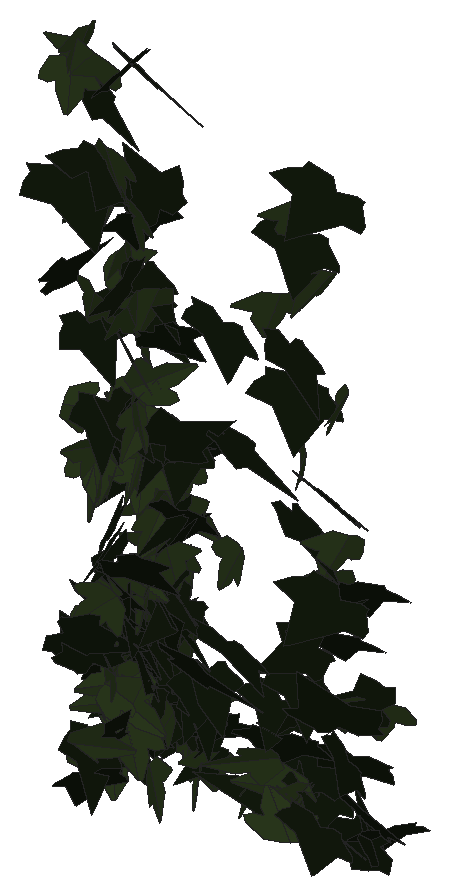
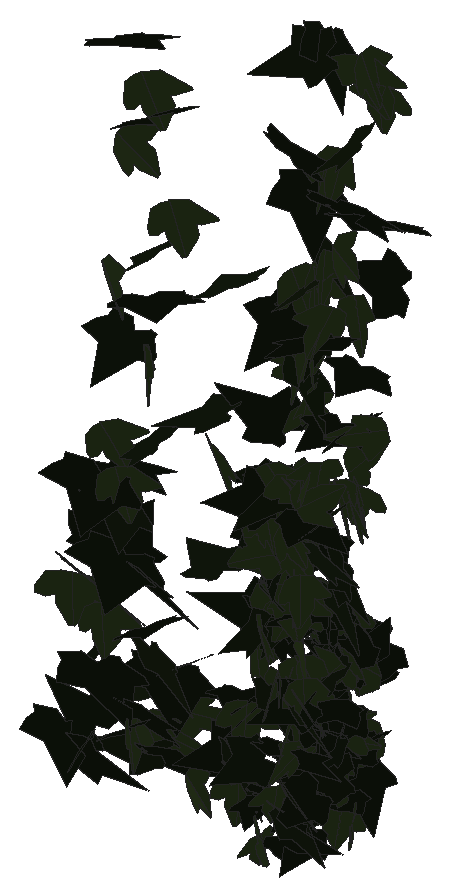
# SketchUp Ruby script. Lengths in millimetres.
U = 1.mm
M = Sketchup.active_model
def pt(a) = Geom::Point3d.new(a.map { |v| v * U })
def face(e, loops, mat)
  f = e.add_face(loops[0].map { |a| pt(a) })
  loops[1..].each { |l| e.add_face(l.map { |a| pt(a) }).erase! }
  f.material = f.back_material = mat if mat
  f
end
# faces: each face lists its corners as indices into pts; further lists are holes
def faces(e, pts, list, mat = nil) = list.each { |f| face(e, (f[0].is_a?(Array) ? f : [f]).map { |l| l.map { |i| pts[i] } }, mat) }
# xy, xz, yz: faces in a plane at the given z, y or x. An outline is a flat list of corners, or four numbers for a rectangle; further outlines are holes
def ring(l) = l.size == 4 ? [[l[0], l[1]], [l[2], l[1]], [l[2], l[3]], [l[0], l[3]]] : l.each_slice(2).to_a
def flat(e, list, mat, &to3) = list.each { |f| face(e, (f[0].is_a?(Array) ? f : [f]).map { |l| ring(l).map { |u, v| to3.(u, v) } }, mat) }
def xy(e, z, list, mat = nil) = flat(e, list, mat) { |x, y| [x, y, z] }
def xz(e, y, list, mat = nil) = flat(e, list, mat) { |x, z| [x, y, z] }
def yz(e, x, list, mat = nil) = flat(e, list, mat) { |y, z| [x, y, z] }
def lines(e, pts, list) = list.each { |a, b| e.add_line(pt(pts[a]), pt(pts[b])) }
# prism: a flat outline (further loops are holes) pulled along v
def prism(e, loops, v, mat = nil)
  f = face(e, loops, mat); d = Geom::Vector3d.new(v.map { |x| x * U })
  f.pushpull(f.normal.samedirection?(d) ? d.length : -d.length)
end
def box(e, o, s, mat = nil) = prism(e, [[o, [o[0] + s[0], o[1], o[2]], [o[0] + s[0], o[1] + s[1], o[2]], [o[0], o[1] + s[1], o[2]]]], [0, 0, s[2]], mat)
def at(x, y, z, deg = 0) = Geom::Transformation.translation(pt([x, y, z])) * Geom::Transformation.rotation(ORIGIN, Z_AXIS, deg.degrees)
def axes(o, x, y, z) = Geom::Transformation.new([*x, 0, *y, 0, *z, 0, *pt(o).to_a, 1])
def part(name) = M.definitions.add(name)
# library, detail: a bought-in or finely detailed component or shape, given as its bounding box
def library(name, o, s) = part(name).tap { |d| box(d.entities, o, s) }
def detail(e, o, s) = box(e.add_group.entities, o, s)
def put(e, d, t, mat = nil) = e.add_instance(d, t).tap { |i| i.material = mat if mat }
def group(e, t, mat = nil) = e.add_group.tap { |g| g.transformation = t; g.material = mat if mat }.entities
root = M.entities
M.materials.add("efeu1").color = [18, 25, 13]
M.materials.add("efeu2").color = [43, 57, 29]
c1 = part("ivyleaf_9")
p = [[39.1,54.8,31.7],[34.5,51.8,30.2],[-5.3,25.2,17.3],[-17.9,28.3,20.9],[-21.6,21.7,17],[-20.2,4.3,5.3],
  [-22.9,-0.3,2.5],[-17.1,-4,-0.6],[-2,-2.1,-1.2],[-0.7,-15.4,-10.1],[16.6,-22.3,-16.7],[21.1,-15.1,-12.5],
  [32.7,-10.7,-11],[46.1,-1.8,-6.6],[30.8,11.2,3.8]]
faces(c1.entities,p,[[0,1,2,3,4,5,6,7,8,9,10,11,12,13,14]],"efeu1")
c2 = part("ivyleaf_10")
p = [[0,12.8,-0.8],[-1.5,51.3,-10.9],[-4.9,51,-11.6],[-13.6,26.5,-7.3],[-13.2,15.9,-4.6],[-21.1,19.3,-7.2],
  [-29.5,16.3,-8.3],[-29.2,8.3,-6.2],[-19.7,-9.8,0.5],[-7.6,-13,4],[1,-12.2,5.8],[-0.4,51.1,-11.1],
  [-1.5,51.1,-10.9],[1,-12.4,5.9],[16.9,-12.4,3.5],[35.1,9.1,-5.1],[35,12.9,-6.1],[20.5,16.4,-4.9],
  [15.8,15,-3.8],[15.3,27.6,-7.1],[12.8,31.3,-7.8]]
faces(c2.entities,p,[[0,1,2,3,4,5,6,7,8,9,10],[11,12,0,13,14,15,16,17,18,19,20]],"efeu2")
put(root,c1,axes([736,1006.8,1673],[-0.48258,0.69438,-0.16098],[-0.11218,-0.23228,-0.77598],[-0.86235,-0.35837,0.19103]))
put(root,c2,axes([717.6,870.9,2505.8],[1.2073,0.09097,0.06116],[0.06582,0.07936,-0.99101],[-0.11642,0.9883,0.07394]))
put(root,c2,axes([725.1,886.3,2544.7],[0.09502,-1.01576,0.19504],[0.05123,-0.19232,-1.0184],[1.26083,0.08436,0.02669]))
put(root,c1,axes([731.4,969.1,1978.9],[-0.96634,0.16266,-0.36138],[0.32603,-0.37717,-0.7555],[-0.35703,-0.78469,0.28823]))
put(root,c2,axes([723.2,924.8,1838.9],[0.90491,-0.52897,-0.04758],[-0.0478,0.027,-0.91103],[0.64619,0.74277,-0.00076]))
put(root,c2,axes([729,903.9,1639.6],[0.31669,-0.47404,-0.71017],[-0.18791,0.70409,-0.52628],[1.02461,0.27564,0.12298]))
put(root,c2,axes([744.6,871.5,2527.6],[-1.64861,0.10035,0.44623],[-0.86974,-0.15074,-0.85322],[-0.03566,-0.96268,0.18012]))
put(root,c2,axes([741.3,969.4,2037.5],[-0.69821,0.05512,-0.68237],[-0.83211,-0.12231,0.56217],[-0.07175,0.88216,0.12058]))
put(root,c1,axes([737.5,997.8,1805.7],[-0.81287,0.5246,-0.03584],[0.02253,-0.03447,-0.84788],[-0.64111,-0.66636,0.01564]))
put(root,c2,axes([726.8,991.4,1824.4],[-0.46572,-0.77141,-0.05585],[0.06616,0.03544,-0.86007],[0.94126,-0.38417,0.03282]))
put(root,c1,axes([715.3,844.8,2258.7],[0.17072,0.92716,-0.37618],[-0.0976,0.38899,0.92897],[1.21678,-0.09888,0.1273]))
put(root,c1,axes([709.9,885.4,2358.7],[-0.72181,-0.79752,-0.36037],[0.82373,0.17043,-0.83269],[1.44765,-0.49463,0.29413]))
put(root,c1,axes([736.3,998.9,1741.5],[-0.89598,-0.36202,0.18741],[-0.19448,-0.10037,-0.81857],[0.45774,-0.75127,0.01905]))
put(root,c1,axes([719.8,982.7,1694.4],[0.6203,0.55737,0.33393],[0.29686,0.22982,-0.75409],[-0.735,0.56321,-0.02275]))
put(root,c2,axes([731.7,923.6,1669],[-0.64135,0.6965,-0.0657],[-0.05246,0.04986,0.87262],[0.85189,0.52744,0.00427]))
put(root,c1,axes([710.8,959,1826.5],[0.4423,-0.69829,0.3383],[0.25011,-0.27393,-0.78513],[0.91298,0.41333,0.05119]))
put(root,c1,axes([712.3,945.4,1703.4],[0.70376,0.08993,0.64163],[0.62061,0.46919,-0.52309],[-0.48953,0.72409,0.25926]))
put(root,c1,axes([742.8,1010.2,1647.9],[-0.14857,-0.20705,-0.77913],[-0.44615,-0.68805,0.24],[-0.87652,0.38531,0.0099]))
put(root,c1,axes([714,955.6,1799.8],[-0.25147,-0.40809,-0.74835],[0.60556,0.56845,-0.4467],[0.84541,-0.52857,0.09737]))
put(root,c1,axes([721.6,939.4,1741.8],[0.91558,-0.22593,-0.36094],[-0.40085,0.158,-0.78206],[0.33045,0.81764,0.05139]))
put(root,c1,axes([743.1,912.1,1894.6],[-0.39537,0.7781,0.31895],[-0.16045,0.29071,-0.84284],[-1.01331,-0.34963,0.00901]))
put(root,c2,axes([716.2,944.2,1835.7],[0.8108,0.05931,0.54121],[0.65816,0.04351,-0.66722],[-0.08963,0.85598,-0.00359]))
put(root,c2,axes([735.8,889.4,2027.4],[0.53517,-0.7577,-0.29504],[-0.14727,0.27084,-0.87502],[0.98101,0.45401,0.0296]))
put(root,c1,axes([731.9,908.8,1764.9],[0.45542,0.7726,0.26468],[0.16634,0.22798,-0.85776],[-0.98236,0.39677,-0.02254]))
put(root,c1,axes([721.4,902.1,2181.3],[-0.45284,-0.47083,-0.70904],[0.67793,0.45188,-0.59095],[0.78654,-0.66055,0.10113]))
put(root,c1,axes([717.5,910.8,2461.5],[0.79664,-0.71391,-0.19548],[-0.02365,0.24409,-0.9562],[0.90272,0.63641,0.14745]))
put(root,c1,axes([720.9,965.6,2021.5],[0.13454,-0.88447,0.1392],[0.16263,-0.12247,-0.88377],[1.08016,0.1286,0.11573]))
put(root,c1,axes([731.7,974.8,1642.6],[0.47381,0.66938,0.24934],[0.1563,0.21394,-0.77388],[-0.85733,0.40894,-0.00328]))
put(root,c2,axes([733,998.4,1745.6],[-0.01133,0.37561,0.74869],[-0.12988,0.74214,-0.37364],[-1.01362,-0.0993,0.03951]))
put(root,c1,axes([709.1,919.4,1827],[0.57125,-0.39976,0.7706],[0.80492,-0.40518,-0.61108],[0.68835,0.80555,0.07506]))
put(root,c2,axes([730.2,959.9,2080.7],[0.58265,0.77237,0.01431],[0.0084,0.01256,-0.90809],[-0.94241,0.47763,0.00075]))
put(root,c2,axes([713.5,896.6,1811],[-0.00894,0.0213,-0.94912],[1.04229,-0.41376,-0.01588],[-0.50507,-0.85421,-0.01597]))
put(root,c2,axes([728.5,927.2,1639.4],[0.88697,0.46011,0.12325],[0.12377,0.07016,-0.86037],[-0.56779,0.73405,0.00498]))
put(root,c1,axes([742.1,987.8,1815.7],[-0.87665,0.277,-0.35839],[0.4005,-0.1446,-0.76996],[-0.38076,-0.78986,0.01527]))
put(root,c1,axes([744.5,971.1,2027.2],[-0.02977,0.36675,-0.81999],[-0.02135,-0.82033,-0.36639],[-1.09568,0.00602,0.02942]))
put(root,c2,axes([751.3,913.8,1724],[-0.17277,-0.06921,0.89006],[-0.64483,-0.71976,-0.14007],[0.87774,-0.5424,0.0723]))
put(root,c1,axes([746.4,904.9,2375.2],[-1.72779,-0.27021,-0.19313],[0.42227,-0.07509,-0.93788],[0.47039,-0.92511,0.13254]))
put(root,c1,axes([743.8,877.4,1786.4],[0.63994,0.20871,0.81274],[-0.99444,-0.10086,0.55197],[0.24309,-0.96204,0.11845]))
put(root,c2,axes([750.3,876.1,2234],[-0.9863,0.21956,0.49643],[-0.58372,0.13238,-0.83773],[-0.31277,-0.93942,-0.00203]))
put(root,c1,axes([728.3,920.7,1665.8],[-0.03432,-0.26209,-0.82208],[0.09454,0.81842,-0.26357],[1.04841,-0.08238,-0.00315]))
put(root,c2,axes([743.8,914.8,1742.7],[-0.10282,0.13445,0.85306],[-0.16595,-0.84848,0.12029],[1.04042,-0.12205,0.10349]))
put(root,c2,axes([735.6,918.3,2323],[0.30207,-0.77973,0.55458],[0.22308,-0.52374,-0.81799],[1.14583,0.30752,0.01305]))
put(root,c2,axes([721.3,877.4,2092.5],[-0.12433,-0.16946,-0.90765],[0.97322,0.44367,-0.1724],[0.56724,-0.79835,0.09685]))
put(root,c2,axes([743.1,882.8,2045.8],[-0.13572,-0.17882,-0.91596],[-0.39439,-0.85796,0.20676],[-1.06808,0.33952,0.04005]))
put(root,c1,axes([744.8,903.1,1927.9],[0.09412,0.37838,0.81761],[0.03316,0.81925,-0.3817],[-1.09863,0.05715,0.05852]))
put(root,c1,axes([748.6,1000.3,1706.5],[-0.86466,0.36783,-0.19995],[0.22377,-0.0806,-0.7984],[-0.45914,-0.73198,-0.01257]))
put(root,c1,axes([723.1,991.5,1809.5],[0.97435,0.01676,0.27768],[0.33253,0.12166,-0.79129],[-0.06786,0.83674,0.10949]))
put(root,c1,axes([733,933.5,1805.6],[-0.18666,-0.79125,-0.28943],[0.08847,0.2807,-0.80573],[1.02407,-0.16847,0.01686]))
put(root,c2,axes([731.3,891,2020.8],[1.05702,0.20621,0.23006],[0.27015,0.06321,-0.89056],[-0.26285,0.8942,0.0099]))
put(root,c2,axes([736,893.7,2000.1],[0.80158,-0.60895,0.23322],[0.22443,-0.14453,-0.89564],[0.76323,0.68205,0.01844]))
put(root,c2,axes([738.8,941.5,1667.1],[-0.10905,0.44318,-0.72072],[-0.03627,-0.72593,-0.44269],[-1.03158,-0.02133,0.09175]))
put(root,c2,axes([744.1,975.5,1938.4],[-0.5166,-0.76141,-0.08895],[0.06216,0.07344,-0.87119],[0.93317,-0.4264,0.00879]))
put(root,c1,axes([749.8,904.2,1922.2],[-0.65855,0.56241,-0.45279],[0.36666,-0.33901,-0.77938],[-0.80093,-0.61762,0.0155]))
put(root,c2,axes([754.8,887.5,1858.6],[0.9417,-0.09258,-0.62262],[-0.73784,0.16407,-0.77417],[0.21291,0.97803,0.07094]))
put(root,c2,axes([745.4,987.5,1772.2],[0.16886,-0.51456,-0.6732],[0.04897,0.68534,-0.51558],[1.03258,0.05164,0.13454]))
put(root,c2,axes([736.6,913.2,1726.6],[0.93062,0.41804,0.17335],[0.1732,0.10154,-0.8696],[-0.52425,0.77563,0.02042]))
put(root,c1,axes([726.9,856,1823],[0.20086,0.2909,-0.99963],[0.42725,0.9376,0.33053],[1.19612,-0.38376,0.0498]))
put(root,c2,axes([741.3,932.4,2250.5],[0.45358,0.76775,0.46826],[-0.00721,0.50878,-0.82949],[-1.0971,0.31407,0.19905]))
put(root,c2,axes([750.3,955.8,1825.5],[-0.09574,-0.85595,-0.12657],[0.02321,0.12607,-0.85742],[1.6466,-0.05154,0.00473]))
put(root,c2,axes([760,885.6,1774.4],[0.39352,-0.132,-0.88914],[-0.57724,0.77827,-0.28718],[0.93243,0.53751,0.19746]))
put(root,c2,axes([743.9,969.3,2070.8],[-0.65818,0.69521,-0.22127],[0.16239,-0.17679,-0.87997],[-0.87514,-0.55566,0.00313]))
put(root,c2,axes([748.5,929.6,1764],[0.22728,-0.80974,0.20425],[0.08657,-0.19317,-0.83052],[1.01515,0.19776,0.02509]))
put(root,c2,axes([761.4,952.1,1839.8],[-0.07546,0.3997,0.77683],[-0.7953,0.49735,-0.3078],[-0.70957,-0.59995,0.26238]))
put(root,c1,axes([760.3,941.1,1735.7],[-0.93968,-0.30032,0.21904],[-0.23196,-0.11474,-0.8259],[0.38968,-0.79251,0.03657]))
put(root,c1,axes([758.3,856,1659.1],[0.28146,0.86352,-0.3889],[-0.24564,-0.3464,-0.88859],[-1.12899,0.29064,0.09638]))
put(root,c2,axes([747,919.3,1742.4],[-0.4042,0.80604,-0.08092],[0.0391,-0.07431,-0.87147],[-0.98753,-0.33285,-0.00139]))
put(root,c2,axes([756.8,959.6,1827.2],[-0.77078,-0.74938,0.15285],[-0.03604,-0.16308,-0.8497],[1.45514,-0.40098,0.05992]))
put(root,c2,axes([753.2,897.7,2014.7],[0.64834,-0.7488,-0.1849],[-0.09965,0.16864,-0.91771],[0.93569,0.5368,0.03038]))
put(root,c2,axes([739.9,959.8,2206.4],[0.14482,-0.36931,0.83747],[0.76007,-0.58605,-0.34675],[0.81804,0.60991,0.17392]))
put(root,c1,axes([750.7,932.8,1771.3],[0.69116,0.66139,0.01987],[0.01602,0.01492,-0.87085],[-0.8071,0.56668,-0.00027]))
put(root,c2,axes([751.6,933.6,1754.1],[0.16921,0.7117,-0.47499],[-0.10863,-0.46658,-0.72509],[-1.03823,0.16481,-0.00155]))
put(root,c2,axes([752.3,1007.2,1697.9],[0.30272,0.78233,-0.00714],[-0.02778,-0.00027,-0.82046],[-0.95408,0.24823,0.02162]))
put(root,c1,axes([755.1,939.8,1684.2],[0.89841,0.27505,-0.37064],[-0.43776,-0.09781,-0.78549],[-0.35418,0.81859,0.03069]))
put(root,c1,axes([747.5,887.5,2088.8],[-0.02216,-0.95704,0.09186],[-0.00737,-0.09176,-0.95721],[1.17294,-0.01865,-0.00428]))
put(root,c1,axes([744,881.2,1683.4],[0.81897,0.69571,0.17028],[-0.15216,-0.11627,0.96673],[0.86047,-0.68272,0.00888]))
put(root,c1,axes([749,874.3,1688.2],[-0.02427,-1.0511,0.16075],[-0.03966,-0.1601,-1.05088],[1.29664,-0.02457,-0.02914]))
put(root,c2,axes([755.9,947.2,1707.3],[0.17231,0.77284,-0.3112],[-0.05984,-0.30738,-0.78561],[-1.01467,0.14937,-0.00652]))
put(root,c1,axes([773.4,995.5,1743],[-0.96985,-0.09923,0.27915],[-0.32044,-0.13375,-0.79552],[0.16721,-0.83186,0.09461]))
put(root,c2,axes([770.5,918.5,1759.8],[0.66931,0.24639,-0.65135],[-0.77824,-0.15483,-0.59586],[-0.34082,0.83741,0.08147]))
put(root,c1,axes([767.8,904.7,1845.9],[0.09704,-0.15827,0.8892],[-0.12332,0.88547,0.16664],[-1.09495,-0.11376,0.06003]))
put(root,c1,axes([747.1,993.7,1724.1],[0.34575,-0.79481,0.06296],[0.0433,-0.05417,-0.84369],[0.97174,0.28521,0.0152]))
put(root,c1,axes([776.4,999.6,1674],[-0.93088,0.22794,0.16029],[-0.21323,-0.02753,-0.79281],[-0.26479,-0.77919,0.0749]))
put(root,c2,axes([757.3,951.6,1689.3],[0.84842,-0.46742,0.16983],[0.16462,-0.10366,-0.83785],[0.58397,0.70832,-0.01054]))
put(root,c2,axes([760.5,930.5,2008.1],[0.77871,-0.65031,0.05837],[0.05505,-0.03751,-0.91119],[0.79466,0.63985,0.00592]))
put(root,c1,axes([743.7,913.7,1860.1],[0.26242,-0.43106,0.73589],[0.62874,-0.539,-0.46637],[0.82902,0.54524,0.12076]))
put(root,c2,axes([765.4,883.6,2410.3],[-1.11871,0.40198,0.01413],[-0.0154,0.00641,-1.00121],[-0.49047,-0.91706,-0.0008]))
put(root,c2,axes([757.1,1022.2,1625.1],[0.46437,-0.65917,-0.25275],[0.16061,-0.21583,0.76115],[-0.84617,-0.40271,0.00577]))
put(root,c2,axes([749.7,851.7,1694.3],[0.3085,-0.03046,1.00775],[0.57542,0.92184,-0.09049],[-1.08712,0.47929,0.23808]))
put(root,c1,axes([748.2,960.3,1803.8],[0.35787,-0.83335,0.10377],[0.05058,-0.10038,-0.85429],[1.59748,0.18987,0.0038]))
put(root,c1,axes([755.1,920.2,1675.2],[0.34521,-0.70848,-0.43848],[-0.08918,0.44019,-0.7584],[1.01258,0.2803,0.0827]))
put(root,c1,axes([777.7,984.6,1804.6],[-0.42966,0.79212,-0.04949],[0.01828,-0.04749,-0.86686],[-0.9681,-0.35245,0.00559]))
put(root,c2,axes([767.1,987.6,1817.4],[0.25119,-0.55728,-0.63968],[0.07148,0.66601,-0.56137],[1.03255,0.08946,0.19447]))
put(root,c1,axes([775.4,935.1,1737.8],[-1.02836,-0.22041,-0.05985],[0.06915,0.01981,-0.87124],[0.26992,-0.84481,-0.00482]))
put(root,c2,axes([769.5,953.2,2041],[-1.04334,-0.32834,-0.08377],[0.0929,0.03539,-0.91604],[0.40283,-0.85856,-0.00572]))
put(root,c1,axes([758.1,932.2,1823.6],[0.06148,-0.69395,0.56336],[0.07548,-0.56019,-0.69558],[1.08786,0.07809,0.01643]))
put(root,c2,axes([765.6,1018,1640.6],[0.14264,0.77451,-0.16715],[-0.02994,-0.16534,-0.78328],[-0.96619,0.11946,-0.00041]))
put(root,c2,axes([770.5,985.5,1815.7],[-0.76645,0.60557,-0.01651],[-0.09559,-0.10481,-0.86287],[-0.73287,-0.61965,0.12982]))
put(root,c2,axes([782.4,953.9,1903.5],[-1.58601,-0.16244,0.23055],[-0.42492,-0.05944,-0.84889],[0.32796,-0.8626,0.01508]))
put(root,c2,axes([771.2,897.6,2291.6],[0.10911,-0.8559,-0.45372],[0.05165,0.45867,-0.85689],[1.18072,0.05903,0.07942]))
put(root,c2,axes([765.2,935.7,2000.8],[1.08167,0.2075,0.01562],[0.01724,0.00815,-0.91056],[-0.25328,0.88672,0.00471]))
put(root,c1,axes([754.7,927.3,1815.7],[0.61988,-0.71757,0.10254],[0.08276,-0.0776,-0.87918],[0.88044,0.5125,0.01045]))
put(root,c1,axes([755.6,894.9,2097],[-0.11151,-0.53308,-0.7751],[0.54874,0.6592,-0.50641],[1.008,-0.41784,0.18994]))
put(root,c1,axes([774.5,994.5,1687.7],[-0.85031,-0.39305,-0.15288],[0.24423,-0.04842,-0.78817],[0.45285,-0.7119,0.13801]))
put(root,c2,axes([776.4,956.8,1983.1],[-0.1567,-0.8267,0.34846],[-0.02924,-0.34873,-0.83616],[1.09412,-0.12772,0.02756]))
put(root,c1,axes([765.3,948,1878.6],[-0.36896,-0.73216,-0.38905],[0.29782,0.31714,-0.78658],[0.96667,-0.37716,0.09384]))
put(root,c2,axes([772.1,906.8,1695.3],[-1.13626,-0.34751,-0.17806],[0.34159,-0.27337,-0.93101],[0.33204,-0.90797,0.34846]))
put(root,c2,axes([776.2,957.7,1809],[-0.5744,0.72127,0.07951],[-0.07077,0.05707,-0.86116],[-0.88245,-0.47406,0.0173]))
put(root,c2,axes([763.3,893.2,1747.3],[0.52275,0.41091,0.72894],[0.52147,0.59656,-0.58754],[-0.87763,0.59922,0.08508]))
put(root,c1,axes([756.5,925,2213.4],[0.21099,-0.7358,-0.55565],[0.36659,0.56579,-0.7108],[1.71611,-0.0304,0.22016]))
put(root,c2,axes([776.1,943.6,1887.8],[-0.88223,-0.38845,-0.33887],[0.40926,0.08864,-0.81747],[0.4775,-0.79367,0.07455]))
put(root,c2,axes([766.7,905.8,1891.2],[-0.58619,-0.19059,-0.76031],[0.94661,0.01081,-0.49305],[0.1356,-0.89934,0.1552]))
put(root,c2,axes([785.1,937.5,1946.2],[0.46374,0.6937,-0.42512],[-0.3296,-0.33498,-0.78818],[-0.93627,0.46152,0.06691]))
put(root,c1,axes([775.9,1004.8,1680.4],[-0.12816,-0.74354,-0.37416],[0.06888,0.36989,-0.75091],[1.01315,-0.1192,0.00372]))
put(root,c2,axes([796.2,958.9,2049.9],[-0.8967,-0.21801,0.51141],[-0.46379,-0.42148,-0.72603],[0.49488,-0.79001,0.24622]))
put(root,c2,axes([780.6,919.1,1866.6],[0.76898,-0.60084,0.28748],[0.27387,-0.18102,-0.87051],[0.76507,0.66871,0.02266]))
put(root,c2,axes([766.2,898.6,1735.9],[0.58096,0.36359,0.82375],[0.83126,0.46369,-0.59855],[-0.71815,0.83085,-0.02644]))
put(root,c2,axes([793,945,1704.4],[0.7065,-0.55595,-0.37786],[-0.29947,0.2894,-0.802],[0.76345,0.628,0.03508]))
put(root,c2,axes([794.6,919.6,1899.5],[0.17275,-0.59992,-0.71314],[-0.20807,0.69246,-0.61639],[1.11774,0.22163,-0.00452]))
put(root,c1,axes([800.4,857.3,2538],[-0.22047,1.07408,0.03515],[0.00749,0.03667,-1.08911],[-1.31106,-0.18041,-0.01214]))
put(root,c1,axes([789.6,946.9,2042.4],[-0.92318,-0.05778,-0.5191],[0.62626,-0.25092,-0.72037],[-0.1176,-0.88267,0.23876]))
put(root,c1,axes([780.2,923.3,1768.4],[0.03122,-0.4334,0.78524],[0.16323,-0.77493,-0.43206],[1.08198,0.12941,0.04253]))
put(root,c1,axes([811.3,855.7,2280.6],[-0.84454,0.82547,-0.08837],[0.08495,-0.05693,-1.07718],[-1.00926,-0.69554,-0.01671]))
put(root,c2,axes([799.5,965,2000.4],[-0.64857,-0.72343,0.14926],[0.04135,-0.20759,-0.88543],[0.90022,-0.51166,0.1482]))
put(root,c2,axes([800.1,902.5,2163.2],[-0.75706,0.6641,0.24978],[-0.181,0.20304,-0.90843],[-0.84647,-0.63737,-0.02914]))
put(root,c1,axes([794.6,869.6,2192.2],[0.98789,-0.24262,-0.57743],[-0.67122,0.17548,-0.84527],[0.36515,0.97893,0.00841]))
put(root,c1,axes([813.5,942.3,1896.6],[-0.92251,0.44442,-0.0887],[-0.00335,-0.17705,-0.8636],[-0.55288,-0.74047,0.15325]))
put(root,c1,axes([813.4,882.3,2141.6],[-0.36809,0.9805,0.14131],[-0.08321,0.1268,-1.0255],[-1.2057,-0.30809,0.02764]))
put(root,c1,axes([792.9,951,2035.8],[0.94759,0.47728,0.09717],[-0.0361,0.22879,-0.8873],[-0.59313,0.74859,0.20924]))
put(root,c2,axes([802.3,890.4,2101.2],[0.41519,0.79523,-0.57393],[-0.29133,-0.52202,-0.86491],[-1.16045,0.41557,0.0118]))
put(root,c1,axes([784.4,916.1,2260.4],[0.41552,-0.91678,-0.02062],[-0.00421,0.02067,-0.94241],[1.74525,0.21832,0.00263]))
put(root,c1,axes([793.9,979.9,1710.9],[0.75945,0.37429,0.41969],[0.27732,0.40518,-0.6985],[-0.62752,0.63205,0.19924]))
put(root,c2,axes([806.5,860.1,2246],[-0.15929,-0.88408,-0.57455],[0.05862,0.57335,-0.89315],[1.285,-0.13575,-0.03047]))
put(root,c2,axes([798.6,972.6,1861.6],[0.71346,-0.57903,0.30021],[0.28797,-0.18799,-0.8224],[0.74178,0.6299,0.03052]))
put(root,c2,axes([807.4,865.3,2369.9],[-1.07875,0.59693,0.11629],[-0.11694,0.06585,-1.06685],[-0.73267,-0.8894,-0.00094]))
put(root,c2,axes([801.7,884.1,2118.4],[-0.32031,0.99795,-0.1218],[0.00983,-0.12379,-1.03164],[-1.22649,-0.26162,0.02354]))
put(root,c1,axes([812.9,870.5,2358.4],[0.39475,0.9691,-0.29244],[-0.10574,-0.27937,-1.02167],[-1.23042,0.33492,-0.00602]))
put(root,c2,axes([816.1,892.4,2250.8],[-0.40945,-0.94792,0.23589],[-0.09946,-0.22137,-1.00558],[1.18758,-0.34537,-0.00289]))
put(root,c1,axes([798.4,860.3,1931.6],[1.15788,0.46168,0.16133],[0.15764,0.10297,-1.05482],[-0.57545,0.95718,0.03566]))
put(root,c1,axes([823,930.1,1966.5],[-0.92456,0.5106,-0.30044],[0.21296,-0.27372,-0.90548],[-0.69069,-0.76789,0.12299]))
put(root,c1,axes([786.4,885.7,2535.7],[1.56328,-0.55445,-0.03092],[0.01851,0.06957,-0.989],[1.0567,0.81903,0.06307]))
put(root,c1,axes([800,965.7,2019],[0.39632,0.2365,0.81663],[0.83261,0.4488,-0.40145],[-0.61856,0.75564,-0.01715]))
put(root,c1,axes([819.9,932,1971.5],[0.77277,0.47937,-0.53501],[-0.63886,-0.18016,-0.78139],[-0.59993,0.80932,0.14295]))
put(root,c1,axes([800.8,929,1821.8],[-0.09953,0.02672,0.92283],[0.46131,-0.84419,0.05787],[1.02752,0.38159,0.06341]))
put(root,c1,axes([811.2,950.5,2043.9],[-0.52822,-0.79055,-0.16017],[0.17222,0.10471,-0.89844],[0.96888,-0.44961,0.07238]))
put(root,c1,axes([825.5,928,1950],[-0.04603,0.94926,0.08622],[0.01002,0.08661,-0.94993],[-1.16282,-0.03683,-0.0116]))
put(root,c2,axes([817.4,917.8,1920.2],[0.31296,0.89548,0.30349],[-0.23601,0.35752,-0.89137],[-1.12912,0.17347,0.27044]))
put(root,c2,axes([818.8,888.7,1665.7],[-0.30111,0.99933,0.07458],[-0.14074,0.04796,-1.02446],[-1.21444,-0.25333,0.10023]))
put(root,c2,axes([799.5,966.9,1952.8],[0.5674,0.0199,0.76704],[0.89614,0.24774,-0.45181],[-0.27061,0.86214,0.11213]))
put(root,c1,axes([831.8,929.6,1866.6],[-1.12905,-0.2025,-0.0311],[0.05154,-0.04781,-0.94571],[0.24457,-0.92474,0.0557]))
put(root,c1,axes([843.5,866.9,2383.4],[0.06844,0.38948,0.99667],[-0.90641,0.73244,-0.2444],[-0.93952,-0.67826,0.3084]))
put(root,c2,axes([825.7,944.8,1813.6],[0.12301,-0.91383,-0.15298],[0.01423,0.15512,-0.91894],[1.13029,0.0975,0.02822]))
put(root,c1,axes([807.7,932.1,1845.7],[0.78766,-0.68494,0.10224],[0.08219,-0.077,-0.94125],[0.84087,0.64912,-0.00377]))
put(root,c1,axes([840.6,965.1,1691.9],[-0.41741,0.77698,0.33054],[-0.14271,0.30959,-0.84881],[-1.02019,-0.36121,-0.0165]))
put(root,c1,axes([818.5,895.3,2206],[0.98087,0.59983,0.14538],[0.16257,0.06442,-1.00271],[-0.73522,0.81449,-0.02776]))
put(root,c2,axes([814.4,879.8,2147.2],[-0.36563,-0.43125,0.90814],[0.56823,0.78024,0.52423],[-1.08694,0.55296,-0.03143]))
put(root,c1,axes([840.9,970.8,1672.3],[-1.01955,0.30864,-0.11911],[0.12555,-0.06502,-0.89052],[-0.38358,-0.84164,0.02512]))
put(root,c2,axes([832.6,959.4,1746.1],[-0.94191,-0.46864,-0.01357],[0.01353,0.00789,-0.90316],[0.57182,-0.77214,-0.00099]))
put(root,c2,axes([825,957.8,1651.1],[0.67582,-0.57966,0.44731],[0.40456,-0.30146,-0.80132],[0.79639,0.64503,0.02747]))
put(root,c2,axes([836.4,966.6,1659.3],[-0.85415,-0.52973,-0.02388],[0.02271,0.01498,-0.87794],[0.64653,-0.70037,-0.00071]))
put(root,c1,axes([818.9,948.1,1850.8],[0.89197,-0.59081,-0.03105],[-0.01079,0.03844,-0.93968],[0.7217,0.73077,0.02432]))
put(root,c1,axes([834.8,951.4,1751.7],[-0.25707,-0.84422,0.28513],[-0.09142,-0.27517,-0.8701],[1.08326,-0.22357,-0.00576]))
put(root,c1,axes([835.7,952,1736.8],[0.13077,-0.91126,0.18831],[0.02163,-0.18752,-0.91753],[1.13502,0.10856,-0.00421]))
put(root,c1,axes([838.5,957.9,1768.8],[-0.38933,-0.70797,-0.46638],[0.43707,0.33903,-0.75979],[0.9374,-0.45212,0.16056]))
put(root,c1,axes([829.5,901,2071.2],[-0.01667,-0.03564,1.02045],[1.24337,-0.06295,0.01145],[0.07626,1.0186,0.03642]))
put(root,c1,axes([834.9,962.6,1697.5],[0.76557,0.2369,0.62073],[0.66712,0.30082,-0.66761],[-0.4604,0.82981,0.06481]))
put(root,c2,axes([890.5,975.4,1645.1],[0.30302,-0.77706,0.26102],[0.09496,-0.25622,-0.7932],[1.5572,0.16683,-0.00242]))
put(root,c1,axes([856.6,886.1,1820.2],[1.04942,-0.42594,0.5652],[0.91245,-0.30224,-0.6955],[0.99081,0.72948,0.04186]))
put(root,c1,axes([887.8,919.9,2229.8],[-0.27938,-0.85586,0.35468],[0.16806,-0.37039,-0.85724],[1.75518,-0.10077,0.13854]))
put(root,c1,axes([883.8,933.8,2084.2],[1.08836,-0.69119,-0.16416],[0.14543,0.26935,-0.86794],[1.34423,0.53049,0.22681]))
put(root,c2,axes([932.4,936.7,1703.3],[0.10691,0.32821,-0.815],[-1.38245,-0.44209,-0.2281],[-0.94072,0.68698,0.24259]))
put(root,c1,axes([951.4,956,1646.4],[-0.90208,0.27178,0.69057],[-1.37421,0.02042,-0.50362],[-0.3263,-0.83734,0.21186]))
put(root,c2,axes([965.5,950.1,1673.7],[-0.47836,0.06871,0.84724],[-1.51036,-0.33552,-0.20822],[0.57963,-0.81757,0.15666]))
put(root,c1,axes([932,962.6,1764.2],[-0.48577,-0.74024,0.3473],[-0.07155,-0.35282,-0.77963],[1.55453,-0.24755,0.07264]))
put(root,c2,axes([941.4,872.2,1987],[1.07267,-0.73561,-0.07785],[-0.02844,0.08653,-0.92582],[1.40755,0.56235,0.04062]))
put(root,c1,axes([918.5,891,1862.7],[0.01968,-0.79594,0.43319],[0.64489,-0.3984,-0.74009],[1.59954,0.17041,0.29306]))
put(root,c1,axes([954.7,932.7,1742.3],[1.0652,0.54688,-0.41967],[-0.61224,-0.2709,-0.78204],[-1.16036,0.64497,0.02737]))
put(root,c1,axes([968.7,947.6,1767.1],[-0.64034,0.78651,0.05578],[-0.02461,0.05513,-0.85539],[-1.50044,-0.33656,-0.00978]))
put(root,c2,axes([967,913.2,2290.3],[-0.83894,-0.83269,0.12018],[0.017,-0.14031,-0.93934],[1.6011,-0.43482,0.07295]))
put(root,c2,axes([972,948.3,1676.5],[-0.16643,-0.76898,0.3322],[-0.05798,-0.33086,-0.77391],[1.5932,-0.09237,0.00654]))
put(root,c1,axes([986.8,967,1702.8],[-1.61659,0.01908,-0.06607],[0.12611,0.00778,-0.84957],[-0.03504,-0.85193,-0.00924]))
put(root,c1,axes([992.6,947.5,1857.5],[-1.55301,0.31104,-0.04551],[0.0934,0.00102,-0.87307],[-0.59093,-0.81727,-0.0184]))
put(root,c2,axes([977.7,971.5,1678.6],[0.0787,-0.78365,-0.3134],[0.04323,0.31469,-0.7839],[1.60571,0.02994,0.03646]))
put(root,c1,axes([966.4,960.2,1804.2],[-0.31176,-0.8486,0.05328],[-0.03316,-0.05089,-0.86423],[1.61789,-0.16456,-0.00745]))
put(root,c2,axes([982.9,906.9,1649.7],[0.92604,0.74159,0.05959],[-0.11561,-0.03137,0.88633],[1.41122,-0.4892,0.0335]))
put(root,c1,axes([956.2,957.7,1654.9],[1.0657,-0.59977,0.31881],[0.53502,-0.17149,-0.81638],[1.17681,0.62111,0.08245]))
put(root,c1,axes([970.8,939.3,2017.2],[0.68111,-0.8283,-0.0312],[-0.0087,0.03201,-0.90227],[1.57752,0.3578,0.00849]))
put(root,c1,axes([986.5,970.2,1676.7],[-0.43053,-0.78199,0.22793],[-0.09757,-0.22242,-0.81396],[1.54713,-0.23163,0.01209]))
put(root,c2,axes([996.9,919.9,2105.2],[0.53786,-0.75864,-0.44209],[0.02889,0.46857,-0.79438],[1.67085,0.23611,0.15605]))
put(root,c1,axes([992,925,2183.4],[-0.82124,-0.81627,-0.11491],[0.06485,0.11193,-0.92305],[1.56751,-0.43229,-0.02201]))
put(root,c1,axes([985.1,915.6,2238.3],[0.26048,-0.9303,0.09037],[0.02734,-0.08923,-0.94032],[1.77868,0.13761,0.00122]))
put(root,c1,axes([1002.3,953.5,1874.6],[1.25598,0.55067,-0.1857],[-0.39259,-0.04073,-0.85383],[-1.034,0.68435,0.09861]))
put(root,c2,axes([1015.1,898.2,2424.1],[-0.7612,-0.86683,0.17718],[-0.04624,-0.18361,-0.95313],[1.68323,-0.39705,0.05394]))
put(root,c2,axes([1020,940.3,1957.3],[-0.75963,-0.80342,0.07175],[-0.01369,-0.07651,-0.89668],[1.5351,-0.39825,0.02751]))
put(root,c1,axes([1011.1,903.8,2387.8],[-0.59811,-0.89178,0.1999],[-0.0177,-0.20826,-0.94368],[1.73926,-0.30879,0.05914]))
put(root,c1,axes([1032.5,959.9,1733.5],[0.73705,0.46714,-0.60312],[-0.88486,-0.39172,-0.60194],[-1.15109,0.60023,0.07654]))
put(root,c2,axes([1027.6,958.3,1796.8],[-0.7217,-0.7726,-0.13833],[0.0752,0.13464,-0.86032],[1.49189,-0.38053,-0.02355]))
put(root,c1,axes([1032.3,924.3,1922.8],[0.36034,0.80387,0.32765],[-0.08227,0.34367,-0.81819],[-1.65009,0.15841,0.11234]))
put(root,c1,axes([1058.1,970.7,1628.5],[-0.73309,0.01188,-0.75127],[-1.39461,-0.19259,0.37266],[-0.31616,0.822,0.09817]))
put(root,c2,axes([1037.9,938.7,2007],[-0.70376,-0.75062,0.3394],[0.01011,-0.37419,-0.82178],[1.5678,-0.33453,0.15765]))
put(root,c2,axes([1039.2,901.5,2345.8],[-0.05291,-0.8184,0.50388],[-0.05336,-0.50318,-0.81882],[1.82834,-0.03837,-0.00932]))
put(root,c1,axes([1051.5,912.4,1952],[-1.40905,-0.54519,0.12969],[-0.21844,-0.06281,-0.91927],[1.04395,-0.749,-0.01731]))
put(root,c1,axes([1031.6,906.2,1668.9],[-0.54056,-0.7347,0.40293],[0.16404,-0.44881,-0.75759],[1.5863,-0.20395,0.21565]))
put(root,c1,axes([1043.3,944,1953.5],[1.24634,0.57749,-0.19298],[-0.30329,-0.11098,-0.87285],[-1.11843,0.67363,0.02164]))
put(root,c2,axes([1048.7,921.6,2191.8],[0.42972,-0.90433,-0.06566],[-0.00219,0.06738,-0.93197],[1.72565,0.22528,0.01517]))
put(root,c1,axes([1055.6,973.2,1620.3],[-0.26954,-0.54631,0.62467],[0.29438,0.60522,0.56436],[-1.55171,0.20971,-0.00144]))
put(root,c1,axes([1044.8,938.5,1741.3],[-0.13935,-0.53236,0.72531],[-0.15369,-0.72088,-0.53726],[1.70543,-0.10846,0.01085]))
put(root,c1,axes([1060.7,894.1,2462.7],[-1.22883,-0.6745,0.29511],[-0.20407,-0.30219,-0.92526],[1.38626,-0.64238,0.12539]))
put(root,c1,axes([1050,881.2,2100.8],[1.59205,0.00069,-0.4552],[-0.84016,0.23361,-0.81088],[0.2114,0.92325,0.20552]))
put(root,c1,axes([1035,966.4,1665.1],[0.21557,-0.43365,0.71974],[0.77442,-0.60711,-0.42983],[1.39922,0.40283,0.12701]))
put(root,c1,axes([1090.8,933.2,1823.7],[-1.19409,0.54168,0.27851],[-0.47325,0.1372,-0.82703],[-1.0582,-0.6726,0.05559]))
put(root,c1,axes([1070.7,968.7,1651.6],[0.51529,0.80063,-0.08179],[-0.0263,-0.08166,-0.84507],[-1.53146,0.27079,-0.01301]))
put(root,c1,axes([1078.6,879.5,1825],[1.09714,0.01295,0.73475],[-1.39408,0.08515,0.5732],[-0.11236,-0.93002,0.06271]))
put(root,c2,axes([1078,949.3,1813.4],[-1.46871,-0.40321,0.02628],[-0.03843,-0.01811,-0.87067],[0.76806,-0.77194,0.00669]))
